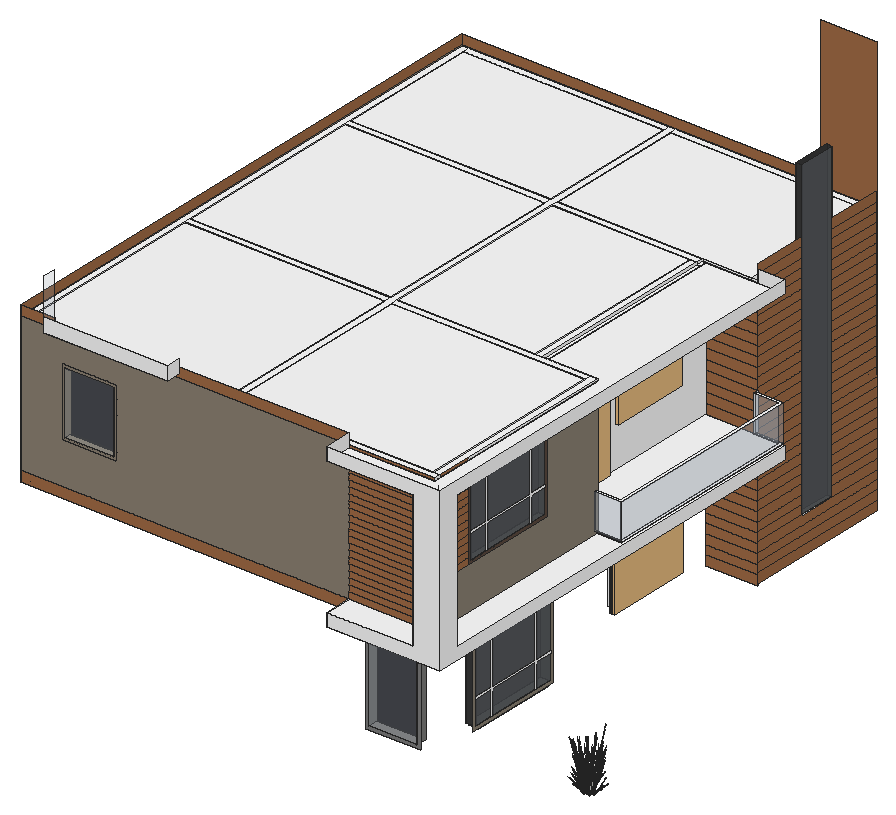
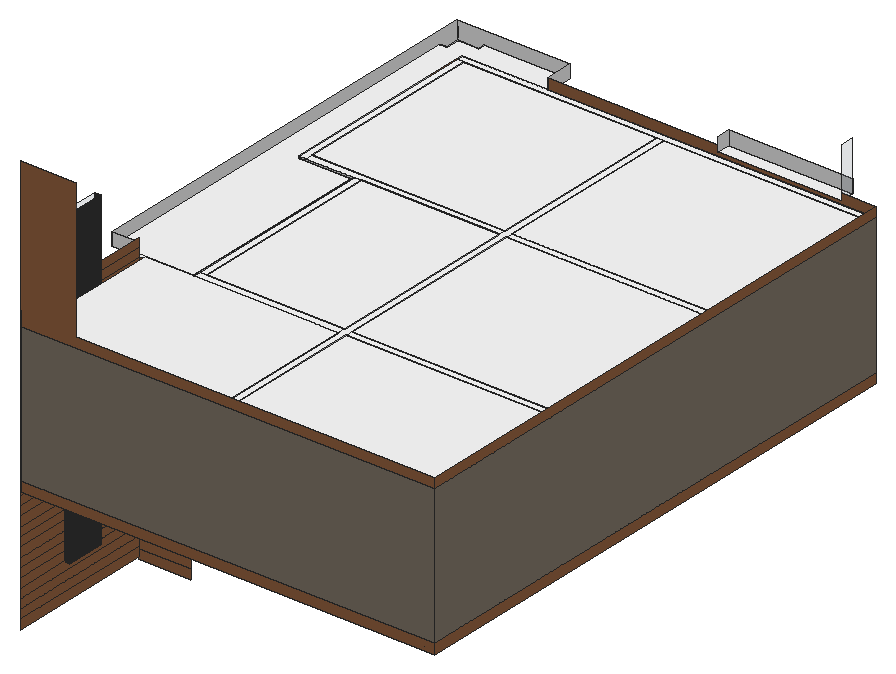
# SketchUp Ruby script. Lengths in inches.
U = 1.inch
M = Sketchup.active_model
def pt(a) = Geom::Point3d.new(a.map { |v| v * U })
def face(e, loops, mat)
  f = e.add_face(loops[0].map { |a| pt(a) })
  loops[1..].each { |l| e.add_face(l.map { |a| pt(a) }).erase! }
  f.material = f.back_material = mat if mat
  f
end
# faces: each face lists its corners as indices into pts; further lists are holes
def faces(e, pts, list, mat = nil) = list.each { |f| face(e, (f[0].is_a?(Array) ? f : [f]).map { |l| l.map { |i| pts[i] } }, mat) }
# xy, xz, yz: faces in a plane at the given z, y or x. An outline is a flat list of corners, or four numbers for a rectangle; further outlines are holes
def ring(l) = l.size == 4 ? [[l[0], l[1]], [l[2], l[1]], [l[2], l[3]], [l[0], l[3]]] : l.each_slice(2).to_a
def flat(e, list, mat, &to3) = list.each { |f| face(e, (f[0].is_a?(Array) ? f : [f]).map { |l| ring(l).map { |u, v| to3.(u, v) } }, mat) }
def xy(e, z, list, mat = nil) = flat(e, list, mat) { |x, y| [x, y, z] }
def xz(e, y, list, mat = nil) = flat(e, list, mat) { |x, z| [x, y, z] }
def yz(e, x, list, mat = nil) = flat(e, list, mat) { |y, z| [x, y, z] }
def lines(e, pts, list) = list.each { |a, b| e.add_line(pt(pts[a]), pt(pts[b])) }
# prism: a flat outline (further loops are holes) pulled along v
def prism(e, loops, v, mat = nil)
  f = face(e, loops, mat); d = Geom::Vector3d.new(v.map { |x| x * U })
  f.pushpull(f.normal.samedirection?(d) ? d.length : -d.length)
end
def box(e, o, s, mat = nil) = prism(e, [[o, [o[0] + s[0], o[1], o[2]], [o[0] + s[0], o[1] + s[1], o[2]], [o[0], o[1] + s[1], o[2]]]], [0, 0, s[2]], mat)
def at(x, y, z, deg = 0) = Geom::Transformation.translation(pt([x, y, z])) * Geom::Transformation.rotation(ORIGIN, Z_AXIS, deg.degrees)
def axes(o, x, y, z) = Geom::Transformation.new([*x, 0, *y, 0, *z, 0, *pt(o).to_a, 1])
def part(name) = M.definitions.add(name)
# library, detail: a bought-in or finely detailed component or shape, given as its bounding box
def library(name, o, s) = part(name).tap { |d| box(d.entities, o, s) }
def detail(e, o, s) = box(e.add_group.entities, o, s)
def put(e, d, t, mat = nil) = e.add_instance(d, t).tap { |i| i.material = mat if mat }
def group(e, t, mat = nil) = e.add_group.tap { |g| g.transformation = t; g.material = mat if mat }.entities
root = M.entities
M.materials.add("Glass_Basic_01").color = [183, 196, 211]
M.materials["Glass_Basic_01"].alpha = 0.23
M.materials.add("I01_Sky_Frost").color = [204, 204, 255]
M.materials.add("LightPink_Translucent").color = [144, 107, 117]
M.materials["LightPink_Translucent"].alpha = 0.75
M.materials.add("M00_Soft_Cloud").color = [255, 255, 255]
M.materials.add("M07_Charcoal_Gleam").color = [58, 58, 58]
M.materials.add("Plaster_04_1K").color = [142, 132, 117]
M.materials.add("ThomThom - Buttons2").color = [40, 40, 43]
M.materials.add("ThomThom - Waistcoat2").color = [127, 127, 126]
M.materials.add("Wood_Floor_12_1K").color = [92, 75, 65]
M.materials.add("Wood_Veneer_15_1K").color = [163, 109, 71]
c1 = part("blade")
p = [[2.15,0.21,22],[0,0.17,0],[0.09,0.45,0],[2.18,0.31,22],[2.29,0.31,22],[0.38,0.45,0],
  [2.48,0.24,33],[2.49,0.24,33],[2.48,0.22,33]]
faces(c1.entities,p,[[0,1,2,3],[4,5,2,3],[6,3,4,7],[8,0,3,6]])
c2 = part("seeds")
p = [[0.3,-0.1,1.38],[-0.01,-0.03,1.59],[-0.01,-0.03,0.03],[0.14,-0.07,-0.07],[0.29,-0.03,3],[0.15,0.01,3.11]]
faces(c2.entities,p,[[0,1,2,3],[1,0,4,5]],"LightPink_Translucent")
c3 = part("blade with seeds")
put(c3.entities,c1,at(0,0,0))
put(c3.entities,c2,axes([2.4,0.25,30.99],[1.5799,-0.05474,1.17369],[-0.12525,1.92788,0.29478],[-0.07173,-0.02425,1.56792]))
c4 = library("mesh-162",[-1607.75,-1245.64,-53.98],[1739.16,1702.88,120.91])
c5 = part("Group9")
put(c5.entities,c4,at(0,0,0))
c6 = library("porta+4",[0.2,-5.42,1.33],[46.55,4.72,83.21])
xy(root,18,[[357,315.98,363,384.98]],"M00_Soft_Cloud")
xy(root,30,[[399,111.98,408,186.98]],"M00_Soft_Cloud")
xy(root,33,[[399,108.98,408,189.98]],"M07_Charcoal_Gleam")
xy(root,33,[[351,63.98,393,72.98]],"ThomThom - Waistcoat2")
xy(root,42,[[403,462.98,408,495.98]],"M07_Charcoal_Gleam")
xy(root,93,[[357,255.98,363,297.98],[357,315.98,363,384.98]],"M00_Soft_Cloud")
xy(root,99,[[399,108.98,408,111.98],[399,111.98,408,186.98],[399,186.98,408,189.98]],"M07_Charcoal_Gleam")
xy(root,99,[[351,63.98,393,72.98]],"ThomThom - Waistcoat2")
xy(root,114.97,[[333.82,39.98,333.82,63.98,408,63.98,408,240.98,399,240.98,399,414.98,432,414.98,432,39.98]],"M00_Soft_Cloud")
xy(root,120,[[57,72.98,228,303.98],[234,72.98,399,234.98],[234,240.98,357,303.98],[363,240.98,399,414.98],[57,303.98,234,309.98],
  [234,303.98,357,309.98],[57,309.98,228,534.98],[234,309.98,357,408.98],[234,414.98,399,534.98]],"M00_Soft_Cloud")
xy(root,126,[[333.82,39.98,408,39.98,408,45.98,426,45.98,426,57.98,432,57.98,432,414.98,363,414.98,363,307.33,360,307.33,360,259.33,363,259.33,363,240.98,408,240.98,408,63.98,333.82,63.98],[54,69.98,228,234.98],[234,69.98,402,69.98,402,72.98,399,72.98,399,234.98,234,234.98],[399,72.98,402,234.98],[402,72.98,408,234.98],
  [54,240.98,228,408.98],[234,240.98,354,408.98],[54,414.98,228,537.98],[234,414.98,402,537.98]],"M00_Soft_Cloud")
xy(root,128,[[408,236.98,432,238.98],[430,238.98,430,410.98,408,410.98,408,412.98,432,412.98,432,238.98]],"M00_Soft_Cloud")
xy(root,129,[[354,262.33,360,304.33]],"M00_Soft_Cloud")
xy(root,160,[[408,236.98,432,236.98,432,412.98,408,412.98,408,410.98,430,410.98,430,238.98,408,238.98]],"M00_Soft_Cloud")
xy(root,161.6875,[[354,315.98,363,384.98]],"M00_Soft_Cloud")
xy(root,165,[[402,102.98,408,183.98]],"M07_Charcoal_Gleam")
xy(root,165,[[87,63.98,129,69.98]],"Plaster_04_1K")
xy(root,219,[[354,262.33,360,304.33]],"M00_Soft_Cloud")
xy(root,219,[[87,63.98,129,69.98]],"Plaster_04_1K")
xy(root,222,[[360,259.33,363,307.33],[354,315.98,363,384.98]],"M00_Soft_Cloud")
xy(root,231,[[402,102.98,408,183.98]],"M07_Charcoal_Gleam")
xy(root,244,[[333.82,39.98,333.82,63.98,408,63.98,408,240.98,363,240.98,363,414.98,432,414.98,432,57.98,426,57.98,426,45.98,408,45.98,408,39.98],[360,240.98,363,408.98],[360,408.98,363,414.98]],"M00_Soft_Cloud")
xy(root,246,[[48,63.98,408,69.98],[48,69.98,54,543.98],[54,69.98,228,234.98],[228,69.98,234,543.98],[234,69.98,402,234.98],
  [402,69.98,408,240.98],[54,234.98,228,240.98],[234,234.98,402,240.98],[54,240.98,228,408.98],[234,240.98,354,408.98],
  [354,240.98,360,408.98],[54,408.98,228,414.98],[234,408.98,360,414.98],[54,414.98,228,537.98],[234,414.98,402,537.98],
  [54,537.98,228,543.98],[234,537.98,402,543.98]],"M00_Soft_Cloud")
xy(root,249,[[78,51.98,186,63.98]],"M00_Soft_Cloud")
xz(root,39.98,[[333.82,114.97,432,114.97,432,255,333.82,255,333.82,244,408,244,408,126,333.82,126]],"M00_Soft_Cloud")
xz(root,45.98,[[408,126,426,244]],"M00_Soft_Cloud")
xz(root,51.98,[[78,249,186,261]],"M00_Soft_Cloud")
xz(root,57.98,[[426,126,432,244]],"M00_Soft_Cloud")
xz(root,63.98,[[351,33,393,99],[87,165,129,219]],"Glass_Basic_01")
xz(root,63.98,[[[48,126,333.82,246],[84,162,132,222]],[[84,162,132,222],[87,165,129,219]]],"Plaster_04_1K")
xz(root,63.98,[[[348,30,396,102],[351,33,393,99]]],"ThomThom - Waistcoat2")
xz(root,63.98,[[48,117,333.82,126],[333.82,126,408,131.45],[333.82,131.45,408,136.91],[333.82,136.91,408,142.36],[333.82,142.36,408,147.82],
  [333.82,147.82,408,153.27],[333.82,153.27,408,158.73],[333.82,158.73,408,164.18],[333.82,164.18,408,169.64],[333.82,169.64,408,175.09],
  [333.82,175.09,408,180.55],[333.82,180.55,408,186],[333.82,186,408,191.45],[333.82,191.45,408,196.91],[333.82,196.91,408,202.36],
  [333.82,202.36,408,207.82],[333.82,207.82,408,213.27],[333.82,213.27,408,218.73],[333.82,218.73,408,224.18],[333.82,224.18,408,229.64],
  [333.82,229.64,408,235.09],[333.82,235.09,408,240.55],[333.82,240.55,408,244],[333.82,244,408,246],[48,246,333.82,246,333.82,255,186,255,186,249,78,249,78,255,48,255]],"Wood_Veneer_15_1K")
xz(root,69.98,[[[54,126,228,246],[87,165,129,219]],[234,126,402,246]],"M00_Soft_Cloud")
xz(root,69.98,[[87,165,129,219]],"ThomThom - Buttons2")
xz(root,72.98,[[351,33,393,99]],"ThomThom - Buttons2")
xz(root,102.98,[[402,165,408,231]],"M07_Charcoal_Gleam")
xz(root,108.98,[[399,33,408,99]],"M07_Charcoal_Gleam")
xz(root,183.98,[[402,165,408,231]],"M07_Charcoal_Gleam")
xz(root,189.98,[[399,33,408,99]],"M07_Charcoal_Gleam")
xz(root,234.98,[[54,126,228,246],[234,126,402,246]],"M00_Soft_Cloud")
xz(root,236.98,[[408,128,432,160]],"Glass_Basic_01")
xz(root,238.98,[[408,128,430,160]],"Glass_Basic_01")
xz(root,240.98,[[54,126,228,246],[234,126,354,246],[360,244,402,246],[402,244,408,246]],"M00_Soft_Cloud")
xz(root,240.98,[[363,126,408,244]],"Plaster_04_1K")
xz(root,259.33,[[360,126,363,222]],"M00_Soft_Cloud")
xz(root,262.33,[[354,129,360,219]],"M00_Soft_Cloud")
xz(root,304.33,[[354,129,360,219]],"M00_Soft_Cloud")
xz(root,307.33,[[360,126,363,222]],"M00_Soft_Cloud")
xz(root,315.98,[[357,18,363,93],[354,161.6875,363,222]],"M00_Soft_Cloud")
xz(root,384.98,[[357,18,363,93],[354,161.6875,363,222]],"M00_Soft_Cloud")
xz(root,408.98,[[54,126,228,246],[234,126,354,246]],"M00_Soft_Cloud")
xz(root,410.98,[[408,128,430,160]],"Glass_Basic_01")
xz(root,412.98,[[408,128,432,160]],"Glass_Basic_01")
xz(root,414.98,[[408,114.97,432,117],[408,117,432,120],[408,120,432,126],[54,126,228,246],[234,126,234,246,360,246,360,244,363,244,363,126],
  [360,244,402,246],[408,244,432,255]],"M00_Soft_Cloud")
xz(root,414.98,[[363,8.21,408,16.42],[363,16.42,408,24.64],[363,24.64,408,32.85],[363,32.85,408,41.0625],[363,41.0625,408,49.27],
  [363,49.27,408,57.49],[363,57.49,408,65.7],[363,65.7,408,73.91],[363,73.91,408,82.125],[363,82.125,408,90.34],
  [363,90.34,408,98.55],[363,98.55,408,106.76],[363,106.76,408,114.97],[363,114.97,399,120],[363,126,408,134.59],
  [363,134.59,408,143.18],[363,143.18,408,151.77],[363,151.77,408,160.36],[363,160.36,408,168.95],[363,168.95,408,177.55],
  [363,177.55,408,186.14],[363,186.14,408,194.73],[363,194.73,408,203.32],[363,203.32,408,211.91],[363,211.91,408,220.5],
  [363,220.5,408,229.09],[363,229.09,408,237.68],[363,237.68,408,244]],"Wood_Veneer_15_1K")
xz(root,462.98,[[403,42,408,314.7]],"M07_Charcoal_Gleam")
xz(root,495.98,[[403,42,408,314.7]],"M07_Charcoal_Gleam")
xz(root,537.98,[[54,126,228,246],[234,126,402,246]],"M00_Soft_Cloud")
xz(root,543.98,[[48,126,408,246]],"Plaster_04_1K")
xz(root,543.98,[[48,117,408,126],[48,246,48,255,360,255,360,375,408,375,408,246]],"Wood_Veneer_15_1K")
yz(root,48,[[63.98,126,543.98,246]],"Plaster_04_1K")
yz(root,48,[[63.98,117,543.98,126],[63.98,246,543.98,255]],"Wood_Veneer_15_1K")
yz(root,54,[[69.98,126,234.98,246],[240.98,126,408.98,246],[414.98,126,537.98,246]],"M00_Soft_Cloud")
yz(root,78,[[51.98,249,63.98,292.64]],"Glass_Basic_01")
yz(root,87,[[63.98,165,69.98,219]],"Plaster_04_1K")
yz(root,129,[[63.98,165,69.98,219]],"Plaster_04_1K")
yz(root,186,[[51.98,249,63.98,261]],"M00_Soft_Cloud")
yz(root,228,[[69.98,126,234.98,246],[240.98,126,408.98,246],[414.98,126,537.98,246]],"M00_Soft_Cloud")
yz(root,234,[[69.98,126,234.98,246],[240.98,126,408.98,246],[414.98,126,537.98,246]],"M00_Soft_Cloud")
yz(root,333.82,[[39.98,114.97,63.98,126],[39.98,244,63.98,255]],"M00_Soft_Cloud")
yz(root,351,[[63.98,33,72.98,99]],"ThomThom - Waistcoat2")
yz(root,354,[[[240.98,126,408.98,246],[315.98,161.6875,384.98,222],[262.33,129,304.33,219]]],"M00_Soft_Cloud")
yz(root,357,[[240.98,117,408.98,120]],"M00_Soft_Cloud")
yz(root,360,[[[259.33,126,307.33,222],[262.33,129,304.33,219]],[240.98,244,408.98,246],[408.98,244,414.98,246]],"M00_Soft_Cloud")
yz(root,363,[[[312.98,15,387.98,96],[315.98,18,384.98,93]],[[240.98,126,259.33,126,259.33,222,307.33,222,307.33,126,414.98,126,414.98,244,240.98,244],[315.98,161.6875,384.98,222]]],"M00_Soft_Cloud")
yz(root,393,[[63.98,33,72.98,99]],"ThomThom - Waistcoat2")
yz(root,399,[[111.98,30,186.98,33]],"I01_Sky_Frost")
yz(root,399,[[240.98,114.97,414.98,120]],"M00_Soft_Cloud")
yz(root,399,[[108.98,33,189.98,99]],"M07_Charcoal_Gleam")
yz(root,402,[[[69.98,126,234.98,246],[102.98,165,183.98,231]]],"M00_Soft_Cloud")
yz(root,402,[[102.98,165,183.98,231]],"M07_Charcoal_Gleam")
yz(root,403,[[462.98,42,495.98,314.7]],"M07_Charcoal_Gleam")
yz(root,408,[[108.98,33,125.48,54],[127.48,33,173.48,54],[175.48,33,189.98,54],[462.98,42.15,495.98,314.7],[108.98,56,125.48,99],
  [127.48,56,173.48,99],[175.48,56,189.98,99],[102.98,165,119.48,186],[121.48,165,167.48,186],[169.48,165,183.98,186],
  [102.98,188,119.48,231],[121.48,188,167.48,231],[169.48,188,183.98,231]],"Glass_Basic_01")
yz(root,408,[[125.48,33,127.48,33,127.48,54,173.48,54,173.48,33,175.48,33,175.48,54,189.98,54,189.98,56,175.48,56,175.48,99,173.48,99,173.48,56,127.48,56,127.48,99,125.48,99,125.48,56,108.98,56,108.98,54,125.48,54],[462.98,42,495.98,42.15],[39.98,126,45.98,244],[410.98,128,412.98,160],[412.98,128,414.98,160],
  [119.48,165,121.48,165,121.48,186,167.48,186,167.48,165,169.48,165,169.48,186,183.98,186,183.98,188,169.48,188,169.48,231,167.48,231,167.48,188,121.48,188,121.48,231,119.48,231,119.48,188,102.98,188,102.98,186,119.48,186],[63.98,244,69.98,246],[99.98,244,240.98,246]],"M00_Soft_Cloud")
yz(root,408,[[[105.98,30,192.98,102],[108.98,33,189.98,99]],[[63.98,126,240.98,126,240.98,244,99.98,244,99.98,234,186.98,234,186.98,162,63.98,162],[236.98,128,238.98,160]]],"Plaster_04_1K")
yz(root,408,[[[99.98,162,186.98,234],[102.98,165,183.98,231]]],"Wood_Floor_12_1K")
yz(root,408,[[414.98,10.05,543.98,18.07],[414.98,18.07,543.98,26.1],[414.98,26.1,543.98,34.125],[414.98,34.125,543.98,34.125,543.98,42.15,495.98,42.15,495.98,42,462.98,42,462.98,42.15,414.98,42.15],[414.98,42.15,462.98,50.17],
  [495.98,42.15,543.98,50.17],[414.98,50.17,462.98,58.2],[495.98,50.17,543.98,58.2],[414.98,58.2,462.98,66.22],[495.98,58.2,543.98,66.22],
  [414.98,66.22,462.98,74.25],[495.98,66.22,543.98,74.25],[414.98,74.25,462.98,82.27],[495.98,74.25,543.98,82.27],[414.98,82.27,462.98,90.3],
  [495.98,82.27,543.98,90.3],[414.98,90.3,462.98,98.32],[495.98,90.3,543.98,98.32],[414.98,98.32,462.98,106.35],[495.98,98.32,543.98,106.35],
  [414.98,106.35,462.98,114.375],[495.98,106.35,543.98,114.375],[414.98,114.375,462.98,122.4],[495.98,114.375,543.98,122.4],[414.98,122.4,462.98,130.42],
  [495.98,122.4,543.98,130.42],[414.98,130.42,462.98,138.45],[495.98,130.42,543.98,138.45],[414.98,138.45,462.98,146.47],[495.98,138.45,543.98,146.47],
  [414.98,146.47,462.98,154.5],[495.98,146.47,543.98,154.5],[414.98,154.5,462.98,162.52],[495.98,154.5,543.98,162.52],[63.98,162,99.98,168],
  [414.98,162.52,462.98,170.55],[495.98,162.52,543.98,170.55],[63.98,168,99.98,174],[414.98,170.55,462.98,178.57],[495.98,170.55,543.98,170.55,543.98,178.57,495.98,178.58],
  [63.98,174,99.98,180],[414.98,178.57,462.98,186.6],[543.98,178.57,543.98,186.6,495.98,186.6,495.98,178.58],[63.98,180,99.98,186],[63.98,186,99.98,192],
  [414.98,186.6,462.98,194.625],[495.98,186.6,543.98,194.625],[63.98,192,99.98,198],[414.98,194.625,462.98,202.65],[495.98,194.625,543.98,202.65],
  [63.98,198,99.98,204],[414.98,202.65,462.98,210.67],[495.98,202.65,543.98,210.67],[63.98,204,99.98,210],[63.98,210,99.98,216],
  [414.98,210.67,462.98,218.7],[495.98,210.67,543.98,218.7],[63.98,216,99.98,222],[414.98,218.7,462.98,226.72],[495.98,218.7,543.98,226.72],
  [63.98,222,99.98,228],[414.98,226.72,462.98,234.75],[495.98,226.72,543.98,234.75],[63.98,228,99.98,234],[63.98,234,99.98,244],
  [414.98,234.75,462.98,242.77],[495.98,234.75,543.98,242.77],[414.98,242.77,462.98,250.8],[495.98,242.77,543.98,250.8],[69.98,244,99.98,246],
  [414.98,250.8,462.98,258.82],[495.98,250.8,543.98,258.82]],"Wood_Veneer_15_1K")
yz(root,426,[[45.98,126,57.98,244]],"M00_Soft_Cloud")
yz(root,430,[[238.98,128,410.98,160]],"Glass_Basic_01")
yz(root,432,[[236.98,128,412.98,160]],"Glass_Basic_01")
yz(root,432,[[39.98,114.97,414.98,114.97,414.98,126,57.98,126,57.98,244,414.98,244,414.98,255,39.98,255]],"M00_Soft_Cloud")
p = [[399,414.98,120],[408,414.98,120],[399,72.98,120],[408,72.98,120],[57,72.98,120],[57,63.98,120],
  [57,534.98,120],[57,543.98,120],[228,72.98,120],[234,72.98,120],[228,534.98,120],[234,534.98,120],
  [399,408.98,120],[408,408.98,120],[399,534.98,120],[408,534.98,120],[363,408.98,120],[357,408.98,120],
  [426,45.98,246],[426,45.98,255],[408,414.98,246.27],[360,414.98,246.27]]
lines(root,p,[[0,1],[2,3],[4,5],[6,7],[8,9],[10,11],[12,13],[14,15],[16,17],[18,19],[20,21]])
put(root,c3,axes([499.02,123.12,7.83],[0.04068,-0.62141,-0.1216],[0.77029,0.01698,-0.67495],[0.29667,0.04317,1.02557]))
put(root,c3,axes([493.25,120.74,7.83],[0.38229,0.5533,-0.1216],[-0.6785,0.2719,-0.67495],[-0.28593,0.073,1.02557]))
put(root,c3,axes([498.94,119.53,7.83],[-0.83505,-0.03027,-0.1216],[0.02282,-0.57322,-0.67495],[0.05801,-0.22077,1.02557]))
put(root,c3,axes([499.875,121.97,7.83],[-0.38229,-0.5533,-0.1216],[0.6785,-0.2719,-0.67495],[0.28593,-0.073,1.02557]))
put(root,c3,axes([495.73,123.82,7.83],[0.74352,-0.28449,-0.1216],[0.36538,0.50492,-0.67495],[0.0981,0.21277,1.02557]))
put(root,c3,axes([494.11,119.59,7.83],[-0.04068,0.62141,-0.1216],[-0.77029,-0.01698,-0.67495],[-0.29667,-0.04317,1.02557]))
put(root,c3,axes([497.5,123.8,7.83],[0.45276,-0.52302,-0.1216],[0.65568,0.30132,-0.67495],[0.22792,0.14777,1.02557]))
put(root,c3,axes([493.28,122.05,7.83],[0.70283,0.33692,-0.1216],[-0.40491,0.48793,-0.67495],[-0.19857,0.16961,1.02557]))
put(root,c3,axes([497.4,118.89,7.83],[-0.74352,0.28449,-0.1216],[-0.36538,-0.50492,-0.67495],[-0.0981,-0.21277,1.02557]))
put(root,c3,axes([499.85,120.66,7.83],[-0.70283,-0.33692,-0.1216],[0.40491,-0.48793,-0.67495],[0.19857,-0.16961,1.02557]))
put(root,c3,axes([498.01,120.71,7.27],[-0.65655,-0.31748,1.38283],[0.69326,-0.49431,0.59665],[0.21183,0.29789,1.33663]))
put(root,c3,axes([492.46,121.29,7.52],[-0.12407,0.07933,1.74944],[0.01055,0.57963,-0.27667],[-0.2844,0.07538,0.14031]))
put(root,c3,axes([501.95,121.11,7.52],[0.10543,-0.09307,1.74944],[-0.13495,-0.57092,-0.27667],[0.26455,-0.10825,0.14031]))
put(root,c3,axes([499.6875,122.75,7.52],[0.16299,-0.01033,1.74944],[0.44707,-0.47471,-0.27667],[0.28992,0.06266,0.14031]))
put(root,c3,axes([499.7,118.62,7.52],[-0.00733,-0.12161,1.74944],[-0.61946,-0.35147,-0.27667],[0.09577,-0.21306,0.14031]))
put(root,c3,axes([492.48,123.45,7.52],[-0.01889,0.12092,1.74944],[0.53598,0.42065,-0.27667],[-0.14032,0.19892,0.14031]))
put(root,c3,axes([495.56,124.95,7.52],[0.09631,0.0984,1.74944],[0.77725,0.03866,-0.27667],[0.07816,0.217,0.14031]))
put(root,c3,axes([496.21,117.57,7.52],[-0.11621,-0.08567,1.74944],[-0.77555,0.05431,-0.27667],[-0.12378,-0.20491,0.14031]))
put(root,c3,axes([493.67,118.51,7.52],[-0.16348,-0.00431,1.74944],[-0.52047,0.43131,-0.27667],[-0.2777,-0.08813,0.14031]))
put(root,c3,axes([493.04,118.88,7.51],[0.05633,0.06098,1.77383],[-0.27155,0.54815,-0.16761],[-0.27501,0.00397,0.31391]))
put(root,c3,axes([495.42,117.29,7.51],[-0.01417,0.07324,1.77383],[-0.6991,0.2658,-0.16761],[-0.20573,-0.13587,0.31391]))
put(root,c3,axes([496.91,124.23,7.51],[0.00225,-0.07398,1.77383],[0.65113,-0.32638,-0.16761],[0.22617,0.1165,0.31391]))
put(root,c3,axes([491.08,121.875,7.51],[0.09697,0.01639,1.77383],[0.29997,0.53988,-0.16761],[-0.1985,0.1417,0.31391]))
put(root,c3,axes([501.58,120.51,7.51],[-0.09924,-0.00464,1.77383],[-0.4121,-0.49725,-0.16761],[0.1655,-0.1635,0.31391]))
put(root,c3,axes([501.4,123.62,7.51],[-0.0687,-0.05349,1.77383],[0.15029,-0.57341,-0.16761],[0.27062,-0.03664,0.31391]))
put(root,c3,axes([492.42,124.69,7.51],[0.0862,-0.03689,1.77383],[0.71245,0.24539,-0.16761],[-0.01674,0.20431,0.31391]))
put(root,c3,axes([499.53,118.18,7.51],[-0.07716,0.04667,1.77383],[-0.75601,-0.15746,-0.16761],[-0.02737,-0.20368,0.31391]))
put(root,c3,axes([494.19,123.18,8.2],[0.83505,0.03027,-0.13498],[-0.02282,0.57322,-0.74919],[-0.05801,0.22077,1.13838]))
put(root,c3,axes([495.62,118.68,8.23],[-0.50709,0.58578,-0.13619],[-0.73436,-0.33748,-0.75594],[-0.25527,-0.1655,1.14864]))
put(root,c3,axes([495.46,118.72,7.53],[0.34533,-0.38816,0.0643],[0.49176,0.22599,0.50621],[-0.15898,-0.12445,0.77189]))
put(root,c3,axes([495.75,124.05,7.53],[-0.55987,0.20767,0.0643],[-0.27403,-0.37869,0.50621],[0.05407,0.16693,0.77189]))
put(root,c3,axes([500.11,120.53,7.53],[0.52161,0.25698,0.0643],[-0.30368,0.36595,0.50621],[0.16723,-0.11831,0.77189]))
put(root,c3,axes([500.18,121.96,7.53],[0.27906,0.41663,0.0643],[-0.50888,0.20393,0.50621],[0.22432,-0.04024,0.77189]))
put(root,c3,axes([493.84,119.48,7.53],[0.03826,-0.46465,0.0643],[0.57772,0.01274,0.50621],[-0.2213,-0.04862,0.77189]))
put(root,c3,axes([499.08,119.33,7.53],[0.62439,0.02847,0.0643],[-0.01712,0.42991,0.50621],[0.06534,-0.16468,0.77189]))
put(root,c3,axes([499.29,123.23,7.53],[-0.03826,0.46465,0.0643],[-0.57772,-0.01274,0.50621],[0.2213,0.04862,0.77189]))
put(root,c3,axes([493.02,122.18,7.53],[-0.52161,-0.25698,0.0643],[0.30368,-0.36595,0.50621],[-0.16723,0.11831,0.77189]))
put(root,c3,axes([497.38,118.66,7.53],[0.55987,-0.20767,0.0643],[0.27403,0.37869,0.50621],[-0.05407,-0.16693,0.77189]))
put(root,c3,axes([492.95,120.75,7.53],[-0.27906,-0.41663,0.0643],[0.50888,-0.20393,0.50621],[-0.22432,0.04024,0.77189]))
put(root,c3,axes([497.67,123.99,7.53],[-0.34533,0.38816,0.0643],[-0.49176,-0.22599,0.50621],[0.15898,0.12445,0.77189]))
put(root,c3,axes([494.05,123.38,7.53],[-0.62439,-0.02847,0.0643],[0.01712,-0.42991,0.50621],[-0.06534,0.16468,0.77189]))
put(root,c3,axes([497.18,118.7,7.53],[0.74868,0.15974,0.48003],[-0.25601,0.52518,0.3958],[-0.04499,-0.20653,0.9933]))
put(root,c3,axes([499.34,123.08,7.53],[-0.56024,0.40262,0.48003],[-0.48318,-0.42758,0.3958],[0.26285,0.07427,0.9933]))
put(root,c3,axes([500.13,121.8125,7.53],[-0.21466,0.55714,0.48003],[-0.70573,-0.19051,0.3958],[0.27753,-0.03348,0.9933]))
put(root,c3,axes([493.17,122.29,7.53],[-0.18844,-0.56237,0.48003],[0.73919,-0.0976,0.3958],[-0.21785,0.13226,0.9933]))
put(root,c3,axes([494.25,123.42,7.53],[-0.54105,-0.41691,0.48003],[0.57458,-0.35956,0.3958],[-0.0998,0.1956,0.9933]))
put(root,c3,axes([498.88,119.29,7.53],[0.54105,0.41691,0.48003],[-0.57458,0.35956,0.3958],[0.0998,-0.1956,0.9933]))
put(root,c3,axes([493,120.9,7.53],[0.21466,-0.55714,0.48003],[0.70573,0.19051,0.3958],[-0.27753,0.03348,0.9933]))
put(root,c3,axes([499.96,120.43,7.53],[0.18844,0.56237,0.48003],[-0.73919,0.0976,0.3958],[0.21785,-0.13226,0.9933]))
put(root,c3,axes([497.81,123.88,7.53],[-0.75571,0.14023,0.48003],[-0.13115,-0.55007,0.3958],[0.17773,0.16212,0.9933]))
put(root,c3,axes([495.96,123.62,7.85],[0.22906,-0.4699,0.35414],[0.66828,0.13705,-0.4572],[0.06128,0.18919,0.87481]))
put(root,c3,axes([497.17,119.09,7.85],[-0.22906,0.4699,0.35414],[-0.66828,-0.13705,-0.4572],[-0.06128,-0.18919,0.87481]))
put(root,c3,axes([498.9,122.88,7.85],[-0.43232,-0.38257,0.35414],[0.49364,-0.36215,-0.4572],[0.25081,0.0551,0.87481]))
put(root,c3,axes([499.61,121.81,7.85],[-0.63144,-0.17046,0.35414],[0.18417,-0.49731,-0.4572],[0.25423,-0.0456,0.87481]))
put(root,c3,axes([494.23,119.83,7.85],[0.43232,0.38257,0.35414],[-0.49364,0.36215,-0.4572],[-0.25081,-0.0551,0.87481]))
put(root,c3,axes([494.52,123.09,7.85],[0.5141,-0.32171,0.35414],[0.48666,0.36734,-0.4572],[-0.07405,0.18664,0.87481]))
put(root,c3,axes([493.625,122.1,7.85],[0.66138,-0.08733,0.35414],[0.17464,0.49921,-0.4572],[-0.18953,0.13408,0.87481]))
put(root,c3,axes([497.5625,123.54,7.85],[-0.11735,-0.49217,0.35414],[0.67083,-0.12996,-0.4572],[0.18018,0.14104,0.87481]))
put(root,c3,axes([499.51,120.61,7.85],[-0.66138,0.08733,0.35414],[-0.17464,-0.49921,-0.4572],[0.18953,-0.13408,0.87481]))
put(root,c3,axes([493.52,120.9,7.85],[0.63144,0.17046,0.35414],[-0.18417,0.49731,-0.4572],[-0.25423,0.0456,0.87481]))
put(root,c3,axes([498.61,119.62,7.85],[-0.5141,0.32171,0.35414],[-0.48666,-0.36734,-0.4572],[0.07405,-0.18664,0.87481]))
put(root,c3,axes([495.57,119.17,7.85],[0.11735,0.49217,0.35414],[-0.67083,0.12996,-0.4572],[-0.18018,-0.14104,0.87481]))
put(root,c3,axes([495.95,124.01,7.86],[-0.74868,-0.15974,0.53283],[0.25601,-0.52518,0.43934],[0.04499,0.20653,1.10256]))
put(root,c3,axes([493.55,119.49,7.89],[0.62747,-0.45094,0.53763],[0.54116,0.47889,0.4433],[-0.29439,-0.08318,1.11249]))
put(root,c3,axes([495.27,118.59,7.89],[0.84639,-0.15705,0.53763],[0.14689,0.61608,0.4433],[-0.19906,-0.18157,1.11249]))
put(root,c3,axes([496.86,125.3,8.45],[0.52505,-0.35054,-0.06488],[0.48109,0.38392,-0.29416],[0.03387,0.10878,0.97024]))
put(root,c3,axes([492.125,123.52,8.45],[0.67048,0.16311,-0.06488],[-0.20625,0.50201,-0.29416],[-0.10966,0.07622,0.97024]))
put(root,c5,axes([362.87,332.96,89.9],[0,0,0.04646],[0,-0.0437,0],[0.03937,0,0]))
put(root,c6,axes([360.24,260.58,124.46],[0,1,0],[-1,0,0],[0,0,1.15408]))
put(root,c5,axes([363.77,334.33,217.5],[0,0,0.03425],[0,-0.04016,0],[0.03937,0,0]))
